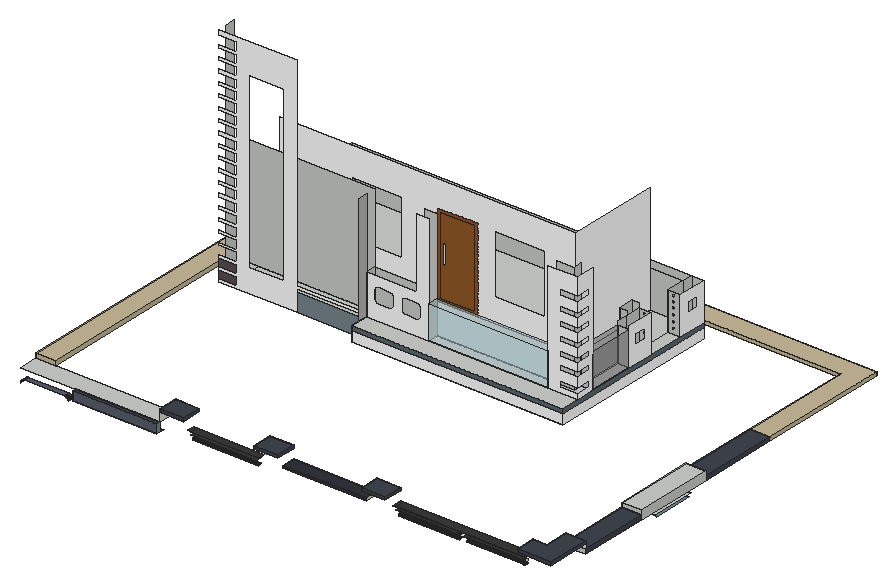
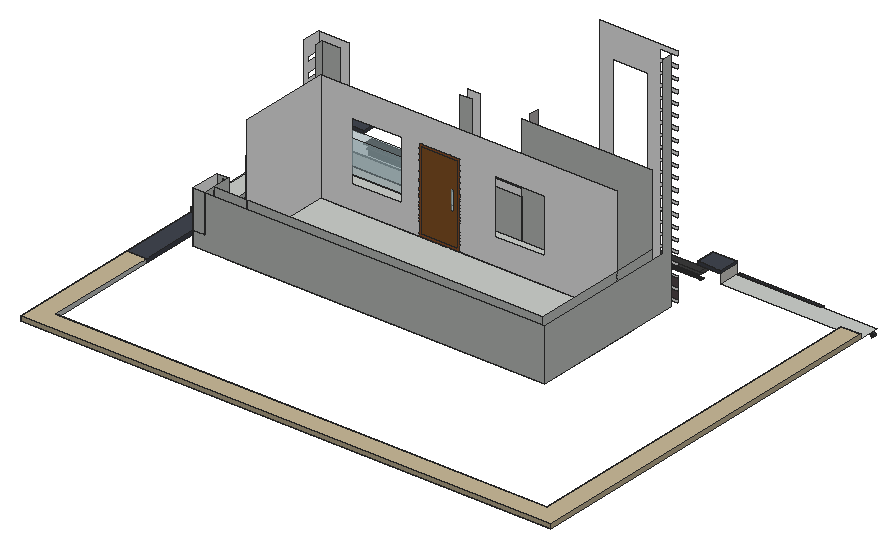
# SketchUp Ruby script. Lengths in inches.
U = 1.inch
M = Sketchup.active_model
def pt(a) = Geom::Point3d.new(a.map { |v| v * U })
def face(e, loops, mat)
  f = e.add_face(loops[0].map { |a| pt(a) })
  loops[1..].each { |l| e.add_face(l.map { |a| pt(a) }).erase! }
  f.material = f.back_material = mat if mat
  f
end
# faces: each face lists its corners as indices into pts; further lists are holes
def faces(e, pts, list, mat = nil) = list.each { |f| face(e, (f[0].is_a?(Array) ? f : [f]).map { |l| l.map { |i| pts[i] } }, mat) }
# xy, xz, yz: faces in a plane at the given z, y or x. An outline is a flat list of corners, or four numbers for a rectangle; further outlines are holes
def ring(l) = l.size == 4 ? [[l[0], l[1]], [l[2], l[1]], [l[2], l[3]], [l[0], l[3]]] : l.each_slice(2).to_a
def flat(e, list, mat, &to3) = list.each { |f| face(e, (f[0].is_a?(Array) ? f : [f]).map { |l| ring(l).map { |u, v| to3.(u, v) } }, mat) }
def xy(e, z, list, mat = nil) = flat(e, list, mat) { |x, y| [x, y, z] }
def xz(e, y, list, mat = nil) = flat(e, list, mat) { |x, z| [x, y, z] }
def yz(e, x, list, mat = nil) = flat(e, list, mat) { |y, z| [x, y, z] }
def lines(e, pts, list) = list.each { |a, b| e.add_line(pt(pts[a]), pt(pts[b])) }
# prism: a flat outline (further loops are holes) pulled along v
def prism(e, loops, v, mat = nil)
  f = face(e, loops, mat); d = Geom::Vector3d.new(v.map { |x| x * U })
  f.pushpull(f.normal.samedirection?(d) ? d.length : -d.length)
end
def box(e, o, s, mat = nil) = prism(e, [[o, [o[0] + s[0], o[1], o[2]], [o[0] + s[0], o[1] + s[1], o[2]], [o[0], o[1] + s[1], o[2]]]], [0, 0, s[2]], mat)
def at(x, y, z, deg = 0) = Geom::Transformation.translation(pt([x, y, z])) * Geom::Transformation.rotation(ORIGIN, Z_AXIS, deg.degrees)
def axes(o, x, y, z) = Geom::Transformation.new([*x, 0, *y, 0, *z, 0, *pt(o).to_a, 1])
def part(name) = M.definitions.add(name)
# library, detail: a bought-in or finely detailed component or shape, given as its bounding box
def library(name, o, s) = part(name).tap { |d| box(d.entities, o, s) }
def detail(e, o, s) = box(e.add_group.entities, o, s)
def put(e, d, t, mat = nil) = e.add_instance(d, t).tap { |i| i.material = mat if mat }
def group(e, t, mat = nil) = e.add_group.tap { |g| g.transformation = t; g.material = mat if mat }.entities
root = M.entities
M.materials.add("[Asphalt New]").color = [89, 79, 82]
M.materials.add("[Basic Tile]").color = [203, 206, 202]
M.materials.add("[Brick Tumbled]").color = [186, 182, 182]
M.materials.add("[Color M00]").color = [255, 255, 255]
M.materials.add("[Color M07]").color = [58, 58, 58]
M.materials.add("[Formica Laminate Dark]").color = [89, 94, 107]
M.materials.add("[Formica Laminate Dark]1").color = [65, 69, 79]
M.materials.add("[Formica Laminate Dark]2").color = [50, 53, 60]
M.materials.add("[Formica Speckled Grey]").color = [120, 135, 142]
M.materials.add("[Formica Speckled Grey]1").color = [94, 105, 111]
M.materials.add("[Quartz Light Brown]").color = [199, 184, 152]
M.materials.add("[Terrazzo Tile Light]").color = [219, 217, 210]
M.materials.add("[Translucent Glass Gray]").color = [128, 128, 128]
M.materials["[Translucent Glass Gray]"].alpha = 0.5
M.materials.add("[Translucent Glass Safety]").color = [204, 235, 244]
M.materials["[Translucent Glass Safety]"].alpha = 0.5
M.materials.add("[Wood Cherry Original]").color = [152, 86, 42]
M.materials.add("[Wood Floor Parquet]").color = [145, 89, 39]
xy(root,168.17,[[171.04,279.43,431.58,289.93],[171.04,289.93,431.58,303.99]],"[Formica Laminate Dark]")
xy(root,175.94,[[26.4,274.68,148.48,289.93]],"[Formica Laminate Dark]")
xy(root,180.91,[[513.6,307.1,716.4,328.82]],"[Color M07]")
xy(root,184.74,[[1333.57,320.24,1344.86,350.55]])
xy(root,184.74,[[1134.85,320.24,1322.28,350.55],[1344.86,320.24,1527,350.55]],"[Color M07]")
xy(root,186.7,[[1639.03,687.97,1649.41,810.49]],"[Formica Speckled Grey]")
xy(root,186.9375,[[795.29,309.57,1053.71,350.55]],"[Basic Tile]")
xy(root,190.375,[[504.35,307.1,513.6,328.82],[513.6,307.1,722.52,328.82]],"[Color M07]")
xy(root,193.9375,[[795.29,309.57,1053.71,350.55]],"[Formica Laminate Dark]2")
xy(root,194.8125,[[0,289.93,431.58,350.55],[0,350.55,0,1547.14,1639.03,1547.14,1639.03,1135.93,1578.42,1135.93,1578.42,1486.52,60.61,1486.52,60.61,350.55],[1578.42,424.2,1639.03,639.97],[1578.42,639.97,1639.03,888.26],[1639.03,679.86,1649.41,818.6],
  [1578.42,888.26,1639.03,1135.93]],"[Basic Tile]")
xy(root,194.8125,[[171.04,279.43,431.58,289.93]],"[Formica Laminate Dark]1")
xy(root,195.17,[[1126.47,320.24,1134.85,350.55],[1134.85,320.24,1535.88,350.55]],"[Color M07]")
xy(root,207.25,[[1578.42,888.26,1639.03,1135.93]],"[Formica Laminate Dark]1")
xy(root,207.25,[[0,350.55,60.61,350.55,60.61,1486.52,1578.42,1486.52,1578.42,1135.93,1639.03,1135.93,1639.03,1547.14,0,1547.14]],"[Quartz Light Brown]")
xy(root,208.1875,[[1578.42,424.2,1639.03,639.97]],"[Formica Laminate Dark]1")
xy(root,221.1875,[[1578.42,639.97,1639.03,888.26]],"[Basic Tile]")
xy(root,222.4375,[[431.58,289.93,504.35,350.55],[1053.71,289.93,1126.47,350.55]])
xy(root,222.4375,[[722.52,289.93,795.29,350.55],[1535.88,289.93,1535.88,350.55,1578.42,350.55,1578.42,424.2,1639.03,424.2,1639.03,289.93]],"[Basic Tile]")
xy(root,231.75,[[431.58,289.93,504.35,350.55],[722.52,289.93,795.29,350.55],[1053.71,289.93,1126.47,350.55],[1535.88,289.93,1639.03,289.93,1639.03,424.2,1578.42,424.2,1578.42,350.55,1535.88,350.55]],"[Formica Laminate Dark]1")
xy(root,349.625,[[716.67,673.46,716.67,730.52,310.19,730.52,310.19,868.79,1290.28,868.79,1290.28,1215.04,1370.47,1215.04,1370.47,673.46],[282.77,730.52,310.19,868.79],[282.77,868.79,310.19,886.125],[310.19,868.79,1262.85,886.125],[1262.85,868.79,1290.28,886.125],
  [282.77,886.125,310.19,1215.04],[310.19,886.125,1262.85,1187.61],[1262.85,886.125,1290.28,1215.04],[310.19,1187.61,1262.85,1215.04]],"[Basic Tile]")
xy(root,393.8125,[[716.67,673.46,1370.47,730.52],[716.67,730.52,909.08,762.76],[909.08,730.52,1278.64,762.76],[1278.64,730.52,1278.64,762.76,1333.54,762.76,1333.54,788.47,1370.47,788.47,1370.47,730.52],[315.01,762.76,1333.54,762.76,1333.54,963.8,1311.73,963.8,1311.73,1012.73,1333.54,1012.73,1333.54,1182.79,1230.77,1182.79,1230.77,898.23,315.01,898.23],
  [1333.54,788.47,1370.47,928.88],[315.01,898.23,1230.77,1182.79],[1333.54,928.88,1370.47,1012.73],[1311.73,963.8,1333.54,1012.73],[1333.54,1012.73,1370.47,1125.19],
  [1333.54,1125.19,1370.47,1215.04]],"[Basic Tile]")
xz(root,279.43,[[171.04,168.17,431.58,194.8125]],"[Formica Laminate Dark]")
xz(root,289.93,[[171.04,168.17,431.58,194.8125]],"[Basic Tile]")
xz(root,289.93,[[431.58,222.4375,504.35,231.75],[722.52,222.4375,795.29,231.75],[1053.71,222.4375,1126.47,231.75],[1535.88,222.4375,1639.03,231.75]],"[Formica Laminate Dark]1")
xz(root,309.57,[[795.29,186.9375,1053.71,193.9375]],"[Formica Laminate Dark]2")
xz(root,350.55,[[431.58,222.4375,504.35,231.75],[722.52,222.4375,795.29,231.75],[1053.71,222.4375,1126.47,231.75],[1535.88,222.4375,1578.42,231.75]],"[Formica Laminate Dark]1")
xz(root,350.55,[[795.29,186.9375,1053.71,193.9375]],"[Formica Laminate Dark]2")
xz(root,350.55,[[0,194.8125,60.61,207.25]],"[Quartz Light Brown]")
xz(root,424.2,[[1578.42,194.8125,1639.03,208.1875]],"[Basic Tile]")
xz(root,424.2,[[1578.42,222.4375,1639.03,231.75]],"[Formica Laminate Dark]1")
xz(root,424.2,[[1578.42,208.1875,1639.03,222.4375]],"[Terrazzo Tile Light]")
xz(root,639.97,[[1578.42,194.8125,1639.03,208.1875],[1578.42,208.1875,1639.03,221.1875]],"[Basic Tile]")
xz(root,673.46,[[716.67,349.625,1370.47,378.99]],"[Color M00]")
xz(root,673.46,[[716.67,378.99,1370.47,393.8125]],"[Formica Speckled Grey]1")
xz(root,703.09,[[282.77,358.58,338.2,383.83],[282.77,391.95,338.2,417.2]],"[Asphalt New]")
xz(root,703.09,[[[282.77,349.625,523.06,349.625,523.06,414.9375,716.67,414.9375,716.67,423.19,523.06,423.19,523.06,1047.125,282.77,1047.125,282.77,1032.02,338.2,1032.02,338.2,1006.77,282.77,1006.77,282.77,997.7,338.2,997.7,338.2,972.45,282.77,972.45,282.77,963.39,338.2,963.39,338.2,938.14,282.77,938.14,282.77,929.08,338.2,929.08,338.2,903.83,282.77,903.83,282.77,894.77,338.2,894.77,338.2,869.52,282.77,869.52,282.77,860.45,338.2,860.45,338.2,835.2,282.77,835.2,282.77,826.14,338.2,826.14,338.2,800.89,282.77,800.89,282.77,791.83,338.2,791.83,338.2,766.58,282.77,766.58,282.77,757.52,338.2,757.52,338.2,732.27,282.77,732.27,282.77,723.2,338.2,723.2,338.2,697.95,282.77,697.95,282.77,688.89,338.2,688.89,338.2,663.64,282.77,663.64,282.77,654.58,338.2,654.58,338.2,629.33,282.77,629.33,282.77,620.27,338.2,620.27,338.2,595.02,282.77,595.02,282.77,585.95,338.2,585.95,338.2,560.7,282.77,560.7,282.77,551.64,338.2,551.64,338.2,526.39,282.77,526.39,282.77,517.33,338.2,517.33,338.2,492.08,282.77,492.08,282.77,483.95,338.2,483.95,338.2,458.7,282.77,458.7,282.77,450.58,338.2,450.58,338.2,425.33,282.77,425.33,282.77,417.2,338.2,417.2,338.2,391.95,282.77,391.95,282.77,383.83,338.2,383.83,338.2,358.58,282.77,358.58],[374.08,421.4,482.58,954.84]]],"[Color M00]")
xz(root,703.09,[[523.06,349.625,716.67,405.57]],"[Formica Speckled Grey]")
xz(root,730.52,[[[716.67,393.8125,909.08,393.8125,909.08,732.375,872.91,732.375,872.91,517.3125,716.67,517.3125],[753.68,440.05,752.03,440.16,750.42,440.48,748.86,441.01,747.38,441.74,746.02,442.65,744.78,443.74,743.69,444.98,742.78,446.35,742.05,447.82,741.52,449.38,741.2,451,741.09,452.64,741.09,475.9,741.2,477.54,741.52,479.16,742.05,480.72,742.78,482.2,743.69,483.56,744.78,484.8,746.02,485.89,747.39,486.8,748.87,487.53,750.43,488.0625,752.04,488.38,753.6875,488.49,788.57,488.49,790.19,488.39,791.78,488.07,793.32,487.55,794.77,486.83,796.12,485.93,797.34,484.86,798.41,483.64,799.31,482.3,800.02,480.84,800.54,479.31,800.86,477.72,800.97,476.1,800.97,452.88,800.86,451.21,800.53,449.5625,799.99,447.97,799.25,446.47,798.32,445.07,797.21,443.8125,795.95,442.71,794.55,441.77,793.05,441.03,791.46,440.49,789.8125,440.16,788.14,440.05],[837.48,440.05,835.83,440.16,834.21,440.48,832.64,441.02,831.16,441.75,829.79,442.67,828.54,443.76,827.45,445,826.53,446.37,825.8,447.85,825.27,449.42,824.95,451.04,824.84,452.69,824.84,476.14,824.95,477.76,825.26,479.34,825.78,480.87,826.5,482.32,827.39,483.66,828.46,484.875,829.67,485.94,831.02,486.84,832.46,487.55,833.99,488.07,835.58,488.39,837.19,488.49,870.38,488.49,872.25,488.37,874.09,488,875.87,487.4,877.55,486.57,879.11,485.53,880.52,484.29,881.76,482.88,882.8,481.32,883.625,479.64,884.23,477.87,884.59,476.03,884.72,474.16,884.72,453.95,884.6,452.14,884.24,450.36,883.66,448.63,882.86,447,881.85,445.49,880.65,444.125,879.28,442.93,877.77,441.92,876.14,441.11,874.42,440.53,872.63,440.17,870.82,440.05]],[1278.64,393.8125,1370.47,393.8125,1370.47,410.47,1314.99,410.47,1314.99,425.22,1370.47,425.22,1370.47,456.66,1314.99,456.66,1314.99,471.41,1370.47,471.41,1370.47,494.79,1314.99,494.79,1314.99,509.54,1370.47,509.54,1370.47,536.91,1314.99,536.91,1314.99,551.66,1370.47,551.66,1370.47,578.29,1314.99,578.29,1314.99,593.04,1370.47,593.04,1370.47,619.47,1314.99,619.47,1314.99,634.22,1370.47,634.22,1370.47,665.22,1314.99,665.22,1314.99,679.97,1370.47,679.97,1370.47,732.375,1278.64,732.375]],"[Color M00]")
xz(root,730.52,[[909.08,393.8125,1278.64,496.0625]],"[Translucent Glass Safety]")
xz(root,762.76,[[315.01,393.8125,716.67,732.375],[716.67,393.8125,716.67,517.3125,872.91,517.3125,872.91,732.375,909.08,732.375,909.08,393.8125],[1278.64,393.8125,1333.54,732.375]],"[Basic Tile]")
xz(root,762.76,[[909.08,393.8125,1278.64,496.0625]],"[Translucent Glass Safety]")
xz(root,788.47,[[1333.54,393.8125,1370.47,499.9375]],"[Basic Tile]")
xz(root,888.26,[[1578.42,194.8125,1639.03,207.25],[1578.42,207.25,1639.03,221.1875]],"[Basic Tile]")
xz(root,898.23,[[[315.01,393.8125,801.1,393.8125,801.1,651.9375,926.47,651.9375,926.47,393.8125,1230.77,393.8125,1230.77,732.375,315.01,732.375],[978.99,466.43,1133.86,648.81],[536.84,474.6,691.07,643.21]]],"[Color M00]")
xz(root,898.23,[[[801.1,393.8125,926.47,651.9375],[809.73,402.45,917.83,643.3]]],"[Wood Cherry Original]")
xz(root,898.23,[[[809.73,402.45,917.83,643.3],[817.84,499.54,826.9,559.11]]],"[Wood Floor Parquet]")
xz(root,928.88,[[1333.54,393.8125,1370.47,499.9375]],"[Basic Tile]")
xz(root,963.8,[[1311.73,393.8125,1333.54,524.8125]],"[Basic Tile]")
xz(root,1012.73,[[1311.73,393.8125,1333.54,524.8125],[[1333.54,393.8125,1370.47,510.75],[1349.2,478.79,1350.53,478.97,1351.77,479.48,1352.83,480.29,1353.64,481.35,1354.15,482.59,1354.33,483.92,1354.15,485.24,1353.64,486.48,1352.83,487.54,1351.77,488.36,1350.53,488.87,1349.2,489.04,1347.875,488.87,1346.64,488.36,1345.58,487.54,1344.76,486.48,1344.25,485.24,1344.08,483.92,1344.25,482.59,1344.76,481.35,1345.58,480.29,1346.64,479.48,1347.875,478.97],[1349.2,423.29,1350.53,423.47,1351.77,423.98,1352.83,424.79,1353.64,425.85,1354.15,427.09,1354.33,428.42,1354.15,429.74,1353.64,430.98,1352.83,432.04,1351.77,432.86,1350.53,433.37,1349.2,433.54,1347.875,433.37,1346.64,432.86,1345.58,432.04,1344.76,430.98,1344.25,429.74,1344.08,428.42,1344.25,427.09,1344.76,425.85,1345.58,424.79,1346.64,423.98,1347.875,423.47],[1349.2,405.1,1350.53,405.28,1351.77,405.79,1352.83,406.61,1353.64,407.67,1354.15,408.9,1354.33,410.23,1354.15,411.56,1353.64,412.79,1352.83,413.85,1351.77,414.67,1350.53,415.18,1349.2,415.35,1347.875,415.18,1346.64,414.67,1345.58,413.85,1344.76,412.79,1344.25,411.56,1344.08,410.23,1344.25,408.9,1344.76,407.67,1345.58,406.61,1346.64,405.79,1347.875,405.28],[1349.2,495.79,1350.53,495.97,1351.77,496.48,1352.83,497.29,1353.64,498.35,1354.15,499.59,1354.33,500.92,1354.15,502.24,1353.64,503.48,1352.83,504.54,1351.77,505.36,1350.53,505.87,1349.2,506.04,1347.875,505.87,1346.64,505.36,1345.58,504.54,1344.76,503.48,1344.25,502.24,1344.08,500.92,1344.25,499.59,1344.76,498.35,1345.58,497.29,1346.64,496.48,1347.875,495.97],[1349.2,461.48,1350.53,461.65,1351.77,462.17,1352.83,462.98,1353.64,464.04,1354.15,465.28,1354.33,466.6,1354.15,467.93,1353.64,469.17,1352.83,470.23,1351.77,471.04,1350.53,471.55,1349.2,471.73,1347.875,471.55,1346.64,471.04,1345.58,470.23,1344.76,469.17,1344.25,467.93,1344.08,466.6,1344.25,465.28,1344.76,464.04,1345.58,462.98,1346.64,462.17,1347.875,461.65],[1349.2,442.67,1350.53,442.84,1351.77,443.35,1352.83,444.17,1353.64,445.23,1354.15,446.47,1354.33,447.79,1354.15,449.12,1353.64,450.35,1352.83,451.42,1351.77,452.23,1350.53,452.74,1349.2,452.92,1347.875,452.74,1346.64,452.23,1345.58,451.42,1344.76,450.35,1344.25,449.12,1344.08,447.79,1344.25,446.47,1344.76,445.23,1345.58,444.17,1346.64,443.35,1347.875,442.84]]],"[Basic Tile]")
xz(root,1125.19,[[[1333.54,393.8125,1370.47,510.75],[1349.2,405.1,1347.875,405.28,1346.64,405.79,1345.58,406.61,1344.76,407.67,1344.25,408.9,1344.08,410.23,1344.25,411.56,1344.76,412.79,1345.58,413.85,1346.64,414.67,1347.875,415.18,1349.2,415.35,1350.53,415.18,1351.77,414.67,1352.83,413.85,1353.64,412.79,1354.15,411.56,1354.33,410.23,1354.15,408.9,1353.64,407.67,1352.83,406.61,1351.77,405.79,1350.53,405.28],[1349.2,478.79,1347.875,478.97,1346.64,479.48,1345.58,480.29,1344.76,481.35,1344.25,482.59,1344.08,483.92,1344.25,485.24,1344.76,486.48,1345.58,487.54,1346.64,488.36,1347.875,488.87,1349.2,489.04,1350.53,488.87,1351.77,488.36,1352.83,487.54,1353.64,486.48,1354.15,485.24,1354.33,483.92,1354.15,482.59,1353.64,481.35,1352.83,480.29,1351.77,479.48,1350.53,478.97],[1349.2,423.29,1347.875,423.47,1346.64,423.98,1345.58,424.79,1344.76,425.85,1344.25,427.09,1344.08,428.42,1344.25,429.74,1344.76,430.98,1345.58,432.04,1346.64,432.86,1347.875,433.37,1349.2,433.54,1350.53,433.37,1351.77,432.86,1352.83,432.04,1353.64,430.98,1354.15,429.74,1354.33,428.42,1354.15,427.09,1353.64,425.85,1352.83,424.79,1351.77,423.98,1350.53,423.47],[1349.2,461.48,1347.875,461.65,1346.64,462.17,1345.58,462.98,1344.76,464.04,1344.25,465.28,1344.08,466.6,1344.25,467.93,1344.76,469.17,1345.58,470.23,1346.64,471.04,1347.875,471.55,1349.2,471.73,1350.53,471.55,1351.77,471.04,1352.83,470.23,1353.64,469.17,1354.15,467.93,1354.33,466.6,1354.15,465.28,1353.64,464.04,1352.83,462.98,1351.77,462.17,1350.53,461.65],[1349.2,442.67,1347.875,442.84,1346.64,443.35,1345.58,444.17,1344.76,445.23,1344.25,446.47,1344.08,447.79,1344.25,449.12,1344.76,450.35,1345.58,451.42,1346.64,452.23,1347.875,452.74,1349.2,452.92,1350.53,452.74,1351.77,452.23,1352.83,451.42,1353.64,450.35,1354.15,449.12,1354.33,447.79,1354.15,446.47,1353.64,445.23,1352.83,444.17,1351.77,443.35,1350.53,442.84],[1349.2,495.79,1347.875,495.97,1346.64,496.48,1345.58,497.29,1344.76,498.35,1344.25,499.59,1344.08,500.92,1344.25,502.24,1344.76,503.48,1345.58,504.54,1346.64,505.36,1347.875,505.87,1349.2,506.04,1350.53,505.87,1351.77,505.36,1352.83,504.54,1353.64,503.48,1354.15,502.24,1354.33,500.92,1354.15,499.59,1353.64,498.35,1352.83,497.29,1351.77,496.48,1350.53,495.97]]],"[Basic Tile]")
xz(root,1135.93,[[1578.42,194.8125,1639.03,207.25]],"[Basic Tile]")
xz(root,1182.79,[[315.01,393.8125,1230.77,510.75],[1230.77,393.8125,1333.54,510.75]],"[Basic Tile]")
xz(root,1215.04,[[282.77,349.625,282.77,510.75,1333.54,510.75,1333.54,393.8125,1370.47,393.8125,1370.47,349.625],[1333.54,393.8125,1370.47,510.75]],"[Basic Tile]")
xz(root,1486.52,[[60.61,194.8125,1578.42,207.25]],"[Quartz Light Brown]")
xz(root,1547.14,[[0,194.8125,1639.03,207.25]],"[Quartz Light Brown]")
yz(root,0,[[350.55,194.8125,1547.14,207.25]],"[Quartz Light Brown]")
yz(root,60.61,[[350.55,194.8125,1486.52,207.25]],"[Quartz Light Brown]")
yz(root,171.04,[[279.43,168.17,289.93,194.8125]],"[Formica Laminate Dark]2")
yz(root,282.77,[[730.52,349.625,730.52,1047.125,762.76,1047.125,762.76,510.75,1215.04,510.75,1215.04,349.625]],"[Basic Tile]")
yz(root,315.01,[[762.76,393.8125,898.23,510.75],[898.23,393.8125,1182.79,510.75]],"[Basic Tile]")
yz(root,431.58,[[289.93,222.4375,350.55,231.75]],"[Formica Laminate Dark]1")
yz(root,431.58,[[279.43,168.17,289.93,194.8125]],"[Formica Speckled Grey]")
yz(root,431.58,[[289.93,194.8125,350.55,222.4375]],"[Terrazzo Tile Light]")
yz(root,504.35,[[289.93,222.4375,350.55,231.75]],"[Formica Laminate Dark]1")
yz(root,716.67,[[673.46,349.625,703.09,393.8125],[703.09,349.625,730.52,393.8125],[730.52,393.8125,762.76,517.3125]],"[Basic Tile]")
yz(root,716.67,[[703.09,393.8125,730.52,732.375]],"[Brick Tumbled]")
yz(root,722.52,[[289.93,222.4375,350.55,231.75]],"[Formica Laminate Dark]1")
yz(root,795.29,[[309.57,186.9375,350.55,193.9375]],"[Basic Tile]")
yz(root,795.29,[[289.93,222.4375,350.55,231.75]],"[Formica Laminate Dark]1")
yz(root,909.08,[[730.52,393.8125,762.76,496.0625]],"[Basic Tile]")
yz(root,1053.71,[[309.57,186.9375,350.55,193.9375]],"[Basic Tile]")
yz(root,1053.71,[[289.93,222.4375,350.55,231.75]],"[Formica Laminate Dark]1")
yz(root,1126.47,[[289.93,222.4375,350.55,231.75]],"[Formica Laminate Dark]1")
yz(root,1134.85,[[337.34,174.52,336.35,174.65,335.43,175.03,334.65,175.63,334.04,176.42,333.66,177.34,333.53,178.33,333.66,179.32,334.04,180.24,334.65,181.03,335.43,181.63,336.35,182.01,337.34,182.14,338.33,182.01,339.25,181.63,340.04,181.03,340.64,180.24,341.02,179.32,341.15,178.33,341.02,177.34,340.64,176.42,340.04,175.63,339.25,175.03,338.33,174.65]])
yz(root,1230.77,[[898.23,393.8125,1182.79,732.375]],"[Color M00]")
yz(root,1278.64,[[730.52,393.8125,762.76,496.0625]],"[Basic Tile]")
yz(root,1311.73,[[963.8,393.8125,1012.73,524.8125]],"[Basic Tile]")
yz(root,1333.54,[[762.76,393.8125,788.47,732.375],[928.88,393.8125,963.8,510.75],[963.8,393.8125,1012.73,510.75],[1125.19,393.8125,1182.79,510.75],[1182.79,393.8125,1215.04,510.75]],"[Basic Tile]")
yz(root,1333.54,[[788.47,393.8125,928.88,499.9375]],"[Translucent Glass Gray]")
yz(root,1370.47,[[673.46,349.625,1215.04,378.99],[730.52,393.8125,788.47,393.8125,788.47,732.375,730.52,732.375,730.52,679.97,774.21,679.97,774.21,665.22,730.52,665.22,730.52,634.22,774.21,634.22,774.21,619.47,730.52,619.47,730.52,593.04,774.21,593.04,774.21,578.29,730.52,578.29,730.52,551.66,774.21,551.66,774.21,536.91,730.52,536.91,730.52,509.54,774.21,509.54,774.21,494.79,730.52,494.79,730.52,471.41,774.21,471.41,774.21,456.66,730.52,456.66,730.52,425.22,774.21,425.22,774.21,410.47,730.52,410.47],[[928.88,393.8125,1012.73,510.75],[951.61,449.17,988.05,477.92]],[[1125.19,393.8125,1215.04,510.75],[1153.55,449.17,1189.99,477.92]]],"[Color M00]")
yz(root,1370.47,[[673.46,378.99,1215.04,393.8125]],"[Formica Speckled Grey]1")
yz(root,1370.47,[[788.47,393.8125,928.88,499.9375]],"[Translucent Glass Gray]")
yz(root,1527,[[337.76,173.35,338.75,173.48,339.67,173.86,340.46,174.47,341.0625,175.26,341.44,176.17,341.57,177.16,341.44,178.15,341.0625,179.07,340.46,179.86,339.67,180.46,338.75,180.84,337.76,180.97,336.77,180.84,335.85,180.46,335.06,179.86,334.46,179.07,334.08,178.15,333.95,177.16,334.08,176.17,334.46,175.26,335.06,174.47,335.85,173.86,336.77,173.48]])
yz(root,1535.88,[[289.93,222.4375,350.55,231.75]],"[Formica Laminate Dark]1")
yz(root,1578.42,[[639.97,194.8125,888.26,221.1875],[1135.93,194.8125,1486.52,207.25]],"[Basic Tile]")
yz(root,1578.42,[[424.2,194.8125,639.97,208.1875],[888.26,194.8125,1135.93,207.25],[350.55,222.4375,424.2,231.75]],"[Formica Laminate Dark]1")
yz(root,1639.03,[[639.97,194.8125,888.26,221.1875]],"[Basic Tile]")
yz(root,1639.03,[[424.2,194.8125,639.97,208.1875],[888.26,194.8125,1135.93,207.25],[289.93,222.4375,424.2,231.75]],"[Formica Laminate Dark]1")
yz(root,1639.03,[[1135.93,194.8125,1547.14,207.25]],"[Quartz Light Brown]")
p = [[716.4,315.95,163.8],[716.4,315.5625,164.74],[513.6,315.5625,164.74],[513.6,315.95,163.8],[716.4,323.05,164.74],[716.4,322.66,163.8],
  [513.6,322.66,163.8],[513.6,323.05,164.74],[1134.85,333.53,164.83],[1134.85,333.66,163.84],[1322.28,333.66,163.84],[1322.28,333.53,164.83],
  [1134.85,341.02,163.84],[1134.85,341.15,164.83],[1322.28,341.15,164.83],[1322.28,341.02,163.84],[1527,333.95,164.29],[1527,334.08,165.27],
  [1344.86,334.08,165.27],[1344.86,333.95,164.29],[1527,341.44,165.27],[1527,341.57,164.29],[1344.86,341.57,164.29],[1344.86,341.44,165.27],
  [13.87,289.93,166.32],[13.54,289.93,164.66],[13.54,274.68,164.66],[13.87,274.68,166.32],[161.32,289.93,164.68],[160.99,289.93,166.34],
  [160.99,274.68,166.34],[161.32,274.68,164.68],[716.4,315.43,165.74],[513.6,315.43,165.74],[716.4,323.18,165.74],[513.6,323.18,165.74],
  [1134.85,333.66,165.82],[1322.28,333.66,165.82],[1134.85,341.02,165.82],[1322.28,341.02,165.82],[1527,334.46,166.19],[1344.86,334.46,166.19],
  [1527,341.0625,166.19],[1344.86,341.0625,166.19],[716.4,315.5625,166.74],[513.6,315.5625,166.74],[716.4,323.05,166.74],[513.6,323.05,166.74],
  [1134.85,334.04,166.74],[1322.28,334.04,166.74],[1134.85,340.64,166.74],[1322.28,340.64,166.74],[1527,335.06,166.98],[1344.86,335.06,166.98],
  [1527,340.46,166.98],[1344.86,340.46,166.98],[14.42,289.93,167.93],[14.42,274.68,167.93],[160.44,289.93,167.94],[160.44,274.68,167.94],
  [716.4,315.95,167.68],[513.6,315.95,167.68],[716.4,322.66,167.68],[513.6,322.66,167.68],[1134.85,334.65,167.53],[1322.28,334.65,167.53],
  [1134.85,340.04,167.53],[1322.28,340.04,167.53],[1527,335.85,167.59],[1344.86,335.85,167.59],[1527,339.67,167.59],[1344.86,339.67,167.59],
  [1134.85,335.43,168.13],[1322.28,335.43,168.13],[1134.85,339.25,168.13],[1322.28,339.25,168.13],[1527,336.77,167.97],[1344.86,336.77,167.97],
  [1527,338.75,167.97],[1344.86,338.75,167.97],[716.4,316.56,168.48],[513.6,316.56,168.48],[716.4,322.04,168.48],[513.6,322.04,168.48],
  [15.17,289.93,169.45],[15.17,274.68,169.45],[159.69,289.93,169.46],[159.69,274.68,169.46],[1527,337.76,168.1],[1344.86,337.76,168.1],
  [1134.85,336.35,168.51],[1322.28,336.35,168.51],[1134.85,338.33,168.51],[1322.28,338.33,168.51],[716.4,317.37,169.09],[513.6,317.37,169.09],
  [716.4,321.24,169.09],[513.6,321.24,169.09],[1134.85,337.34,168.64],[1322.28,337.34,168.64],[716.4,318.3,169.48],[513.6,318.3,169.48],
  [716.4,320.31,169.48],[513.6,320.31,169.48],[16.11,289.93,170.86],[16.11,274.68,170.86],[158.75,289.93,170.87],[158.75,274.68,170.87],
  [716.4,319.3,169.61],[513.6,319.3,169.61],[17.23,289.93,172.14],[17.23,274.68,172.14],[157.64,289.93,172.14],[157.64,274.68,172.14],
  [18.5,289.93,173.25],[18.5,274.68,173.25],[156.36,289.93,173.26],[156.36,274.68,173.26],[19.91,289.93,174.2],[19.91,274.68,174.2],
  [154.96,289.93,174.2],[154.96,274.68,174.2],[1527,337.76,173.35],[1527,336.77,173.48],[1344.86,336.77,173.48],[1344.86,337.76,173.35],
  [1527,338.75,173.48],[1344.86,338.75,173.48],[1527,335.85,173.86],[1344.86,335.85,173.86],[1527,339.67,173.86],[1344.86,339.67,173.86],
  [1527,335.06,174.47],[1344.86,335.06,174.47],[1527,340.46,174.47],[1344.86,340.46,174.47],[21.4375,289.93,174.95],[21.4375,274.68,174.95],
  [153.4375,289.93,174.95],[153.4375,274.68,174.95],[1527,334.46,175.26],[1344.86,334.46,175.26],[1134.85,336.35,174.65],[1134.85,337.34,174.52],
  [1322.28,337.34,174.52],[1322.28,336.35,174.65],[1134.85,338.33,174.65],[1322.28,338.33,174.65],[1527,341.0625,175.26],[1344.86,341.0625,175.26],
  [1134.85,335.43,175.03],[1322.28,335.43,175.03],[1134.85,339.25,175.03],[1322.28,339.25,175.03],[23.04,289.93,175.49],[23.04,274.68,175.49],
  [151.83,289.93,175.49],[151.83,274.68,175.49],[1134.85,334.65,175.63],[1322.28,334.65,175.63],[1134.85,340.04,175.63],[1322.28,340.04,175.63],
  [1527,334.08,176.17],[1344.86,334.08,176.17],[1527,341.44,176.17],[1344.86,341.44,176.17],[24.71,289.93,175.82],[24.71,274.68,175.82],
  [150.17,289.93,175.82],[150.17,274.68,175.82],[1134.85,334.04,176.42],[1322.28,334.04,176.42],[1134.85,340.64,176.42],[1322.28,340.64,176.42],
  [26.4,289.93,175.94],[26.4,274.68,175.94],[148.48,289.93,175.94],[148.48,274.68,175.94],[1527,333.95,177.16],[1344.86,333.95,177.16],
  [1527,341.57,177.16],[1344.86,341.57,177.16],[1134.85,333.66,177.34],[1322.28,333.66,177.34],[1134.85,341.02,177.34],[1322.28,341.02,177.34],
  [1527,334.08,178.15],[1344.86,334.08,178.15],[1527,341.44,178.15],[1344.86,341.44,178.15],[1134.85,333.53,178.33],[1322.28,333.53,178.33],
  [1134.85,341.15,178.33],[1322.28,341.15,178.33],[1527,334.46,179.07],[1344.86,334.46,179.07],[1527,341.0625,179.07],[1344.86,341.0625,179.07],
  [1134.85,333.66,179.32],[1322.28,333.66,179.32],[1134.85,341.02,179.32],[1322.28,341.02,179.32],[1527,335.06,179.86],[1344.86,335.06,179.86],
  [1527,340.46,179.86],[1344.86,340.46,179.86],[1134.85,334.04,180.24],[1322.28,334.04,180.24],[1134.85,340.64,180.24],[1322.28,340.64,180.24],
  [1527,335.85,180.46],[1344.86,335.85,180.46],[1527,339.67,180.46],[1344.86,339.67,180.46],[1134.85,334.65,181.03],[1322.28,334.65,181.03],
  [1134.85,340.04,181.03],[1322.28,340.04,181.03],[1527,336.77,180.84],[1344.86,336.77,180.84],[1527,338.75,180.84],[1344.86,338.75,180.84],
  [1527,337.76,180.97],[1344.86,337.76,180.97],[1134.85,335.43,181.63],[1322.28,335.43,181.63],[1134.85,339.25,181.63],[1322.28,339.25,181.63],
  [1134.85,336.35,182.01],[1322.28,336.35,182.01],[1134.85,338.33,182.01],[1322.28,338.33,182.01],[1134.85,337.34,182.14],[1322.28,337.34,182.14],
  [310.19,730.52,349.625],[310.19,730.52,393.8125]]
faces(root,p,[[0,1,2,3],[4,5,6,7],[8,9,10,11],[12,13,14,15],[16,17,18,19],[20,21,22,23],[1,32,33,2],[34,4,7,35],
  [36,8,11,37],[13,38,39,14],[17,40,41,18],[42,20,23,43],[32,44,45,33],[46,34,35,47],[48,36,37,49],[38,50,51,39],
  [40,52,53,41],[54,42,43,55],[44,60,61,45],[62,46,47,63],[64,48,49,65],[50,66,67,51],[52,68,69,53],[70,54,55,71],
  [72,64,65,73],[66,74,75,67],[68,76,77,69],[78,70,71,79],[60,80,81,61],[82,62,63,83],[76,88,89,77],[88,78,79,89],
  [90,72,73,91],[74,92,93,75],[80,94,95,81],[96,82,83,97],[98,90,91,99],[92,98,99,93],[94,100,101,95],[102,96,97,103],
  [100,108,109,101],[108,102,103,109],[122,123,124,125],[126,122,125,127],[123,128,129,124],[130,126,127,131],[128,132,133,129],[134,130,131,135],
  [132,140,141,133],[142,143,144,145],[143,146,147,144],[148,134,135,149],[150,142,145,151],[146,152,153,147],[158,150,151,159],[152,160,161,153],
  [140,162,163,141],[164,148,149,165],[170,158,159,171],[160,172,173,161],[162,178,179,163],[180,164,165,181],[182,170,171,183],[172,184,185,173],
  [178,186,187,179],[188,180,181,189],[190,182,183,191],[184,192,193,185],[186,194,195,187],[196,188,189,197],[198,190,191,199],[192,200,201,193],
  [194,202,203,195],[204,196,197,205],[206,198,199,207],[200,208,209,201],[202,210,211,203],[212,204,205,213],[214,206,207,215],[208,216,217,209],
  [210,218,219,211],[220,212,213,221],[218,222,223,219],[222,220,221,223],[224,214,215,225],[216,226,227,217],[228,224,225,229],[226,230,231,227],
  [232,228,229,233],[230,232,233,231]],"[Color M07]")
faces(root,p,[[24,25,26,27],[28,29,30,31],[56,24,27,57],[29,58,59,30],[84,56,57,85],[58,86,87,59],[104,84,85,105],[86,106,107,87],
  [110,104,105,111],[106,112,113,107],[114,110,111,115],[112,116,117,113],[118,114,115,119],[116,120,121,117],[136,118,119,137],[120,138,139,121],
  [154,136,137,155],[138,156,157,139],[166,154,155,167],[156,168,169,157],[174,166,167,175],[168,176,177,169]],"[Formica Laminate Dark]")
lines(root,p,[[234,235]])
